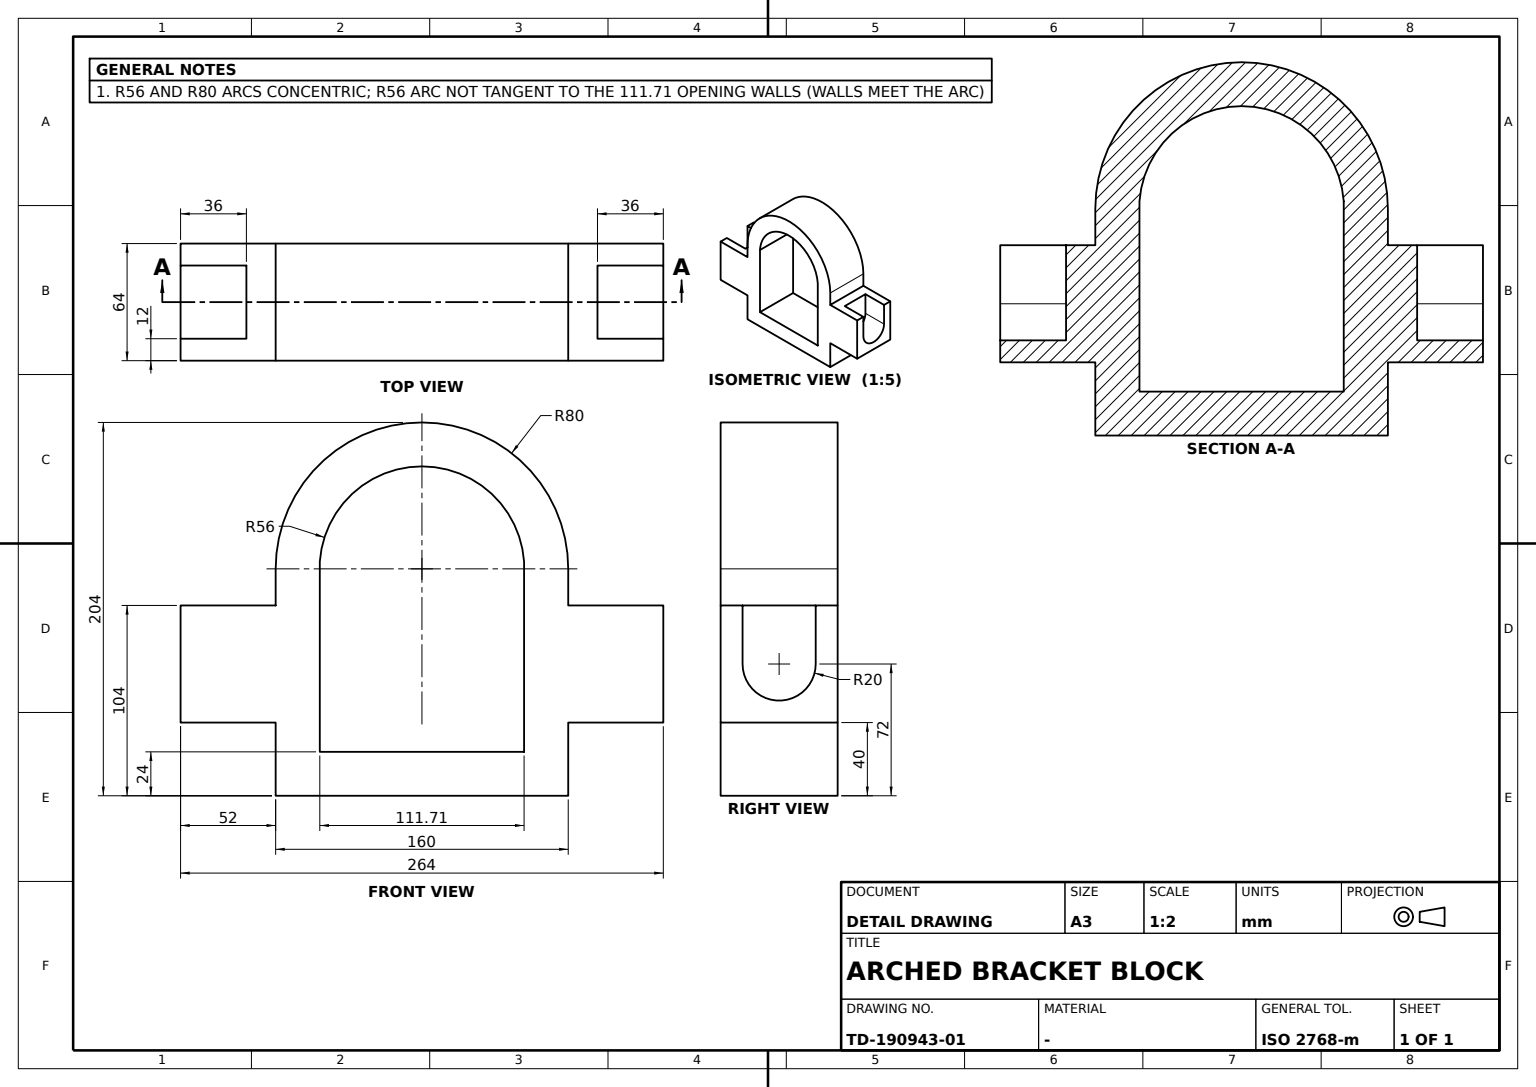
ISO-10303-21;
HEADER;
FILE_DESCRIPTION((''),'2;1');
FILE_NAME('','',(''),(''),'','','');
FILE_SCHEMA(('AUTOMOTIVE_DESIGN'));
ENDSEC;
DATA;
#1=APPLICATION_CONTEXT('');
#2=PRODUCT_CONTEXT('',#1,'mechanical');
#3=PRODUCT('','','',(#2));
#4=PRODUCT_DEFINITION_FORMATION('','',#3);
#5=PRODUCT_DEFINITION_CONTEXT('',#1,'design');
#6=PRODUCT_DEFINITION('','',#4,#5);
#7=PRODUCT_DEFINITION_SHAPE('','',#6);
#8=(LENGTH_UNIT()NAMED_UNIT(*)SI_UNIT(.MILLI.,.METRE.));
#9=(NAMED_UNIT(*)PLANE_ANGLE_UNIT()SI_UNIT($,.RADIAN.));
#10=(NAMED_UNIT(*)SI_UNIT($,.STERADIAN.)SOLID_ANGLE_UNIT());
#11=UNCERTAINTY_MEASURE_WITH_UNIT(LENGTH_MEASURE(0.005),#8,'distance_accuracy_value','');
#12=(GEOMETRIC_REPRESENTATION_CONTEXT(3)GLOBAL_UNCERTAINTY_ASSIGNED_CONTEXT((#11))GLOBAL_UNIT_ASSIGNED_CONTEXT((#8,#9,#10))REPRESENTATION_CONTEXT('',''));
#13=CARTESIAN_POINT('',(20.,-96.,-52.));
#14=VERTEX_POINT('',#13);
#15=CARTESIAN_POINT('',(-20.,-96.,-52.));
#16=VERTEX_POINT('',#15);
#17=CARTESIAN_POINT('',(0.,-96.,-52.));
#18=DIRECTION('',(0.,1.,0.));
#19=DIRECTION('',(0.,0.,1.));
#20=AXIS2_PLACEMENT_3D('',#17,#18,#19);
#21=CIRCLE('',#20,20.);
#22=EDGE_CURVE('',#14,#16,#21,.T.);
#23=ORIENTED_EDGE('',*,*,#22,.T.);
#24=CARTESIAN_POINT('',(-20.,-132.,-52.));
#25=VERTEX_POINT('',#24);
#26=CARTESIAN_POINT('',(-20.,114.,-52.));
#27=VECTOR('',#18,1000.);
#28=LINE('',#26,#27);
#29=EDGE_CURVE('',#25,#16,#28,.T.);
#30=ORIENTED_EDGE('',*,*,#29,.F.);
#31=CARTESIAN_POINT('',(20.,-132.,-52.));
#32=VERTEX_POINT('',#31);
#33=CARTESIAN_POINT('',(0.,-132.,-52.));
#34=DIRECTION('',(0.,-1.,0.));
#35=DIRECTION('',(0.,0.,-1.));
#36=AXIS2_PLACEMENT_3D('',#33,#34,#35);
#37=CIRCLE('',#36,20.);
#38=EDGE_CURVE('',#32,#25,#37,.F.);
#39=ORIENTED_EDGE('',*,*,#38,.F.);
#40=CARTESIAN_POINT('',(20.,114.,-52.));
#41=LINE('',#40,#27);
#42=EDGE_CURVE('',#32,#14,#41,.T.);
#43=ORIENTED_EDGE('',*,*,#42,.T.);
#44=EDGE_LOOP('',(#23,#30,#39,#43));
#45=FACE_BOUND('',#44,.T.);
#46=CARTESIAN_POINT('',(0.,114.,-52.));
#47=DIRECTION('',(-1.,0.,0.));
#48=AXIS2_PLACEMENT_3D('',#46,#18,#47);
#49=CYLINDRICAL_SURFACE('',#48,20.);
#50=ADVANCED_FACE('',(#45),#49,.F.);
#51=CARTESIAN_POINT('',(32.,132.,-84.));
#52=VERTEX_POINT('',#51);
#53=CARTESIAN_POINT('',(32.,80.,-84.));
#54=VERTEX_POINT('',#53);
#55=CARTESIAN_POINT('',(32.,-132.,-84.));
#56=VECTOR('',#34,1000.);
#57=LINE('',#55,#56);
#58=EDGE_CURVE('',#52,#54,#57,.T.);
#59=ORIENTED_EDGE('',*,*,#58,.T.);
#60=CARTESIAN_POINT('',(-32.,80.,-84.));
#61=VERTEX_POINT('',#60);
#62=CARTESIAN_POINT('',(0.,80.,-84.));
#63=DIRECTION('',(1.,0.,0.));
#64=VECTOR('',#63,1000.);
#65=LINE('',#62,#64);
#66=EDGE_CURVE('',#61,#54,#65,.T.);
#67=ORIENTED_EDGE('',*,*,#66,.F.);
#68=CARTESIAN_POINT('',(-32.,132.,-84.));
#69=VERTEX_POINT('',#68);
#70=CARTESIAN_POINT('',(-32.,-132.,-84.));
#71=LINE('',#70,#56);
#72=EDGE_CURVE('',#69,#61,#71,.T.);
#73=ORIENTED_EDGE('',*,*,#72,.F.);
#74=CARTESIAN_POINT('',(0.,132.,-84.));
#75=LINE('',#74,#64);
#76=EDGE_CURVE('',#69,#52,#75,.T.);
#77=ORIENTED_EDGE('',*,*,#76,.T.);
#78=EDGE_LOOP('',(#59,#67,#73,#77));
#79=FACE_BOUND('',#78,.T.);
#80=CARTESIAN_POINT('',(0.,-132.,-84.));
#81=AXIS2_PLACEMENT_3D('',#80,#35,#18);
#82=PLANE('',#81);
#83=ADVANCED_FACE('',(#79),#82,.T.);
#84=CARTESIAN_POINT('',(-32.,-80.,-84.));
#85=VERTEX_POINT('',#84);
#86=CARTESIAN_POINT('',(-32.,-80.,-124.));
#87=VERTEX_POINT('',#86);
#88=CARTESIAN_POINT('',(-32.,-80.,0.));
#89=VECTOR('',#35,1000.);
#90=LINE('',#88,#89);
#91=EDGE_CURVE('',#85,#87,#90,.T.);
#92=ORIENTED_EDGE('',*,*,#91,.T.);
#93=CARTESIAN_POINT('',(32.,-80.,-124.));
#94=VERTEX_POINT('',#93);
#95=CARTESIAN_POINT('',(0.,-80.,-124.));
#96=LINE('',#95,#64);
#97=EDGE_CURVE('',#87,#94,#96,.T.);
#98=ORIENTED_EDGE('',*,*,#97,.T.);
#99=CARTESIAN_POINT('',(32.,-80.,-84.));
#100=VERTEX_POINT('',#99);
#101=CARTESIAN_POINT('',(32.,-80.,0.));
#102=LINE('',#101,#89);
#103=EDGE_CURVE('',#100,#94,#102,.T.);
#104=ORIENTED_EDGE('',*,*,#103,.F.);
#105=CARTESIAN_POINT('',(0.,-80.,-84.));
#106=LINE('',#105,#64);
#107=EDGE_CURVE('',#85,#100,#106,.T.);
#108=ORIENTED_EDGE('',*,*,#107,.F.);
#109=EDGE_LOOP('',(#92,#98,#104,#108));
#110=FACE_BOUND('',#109,.T.);
#111=CARTESIAN_POINT('',(0.,-80.,0.));
#112=AXIS2_PLACEMENT_3D('',#111,#34,#35);
#113=PLANE('',#112);
#114=ADVANCED_FACE('',(#110),#113,.T.);
#115=CARTESIAN_POINT('',(20.,96.,-52.));
#116=VERTEX_POINT('',#115);
#117=CARTESIAN_POINT('',(-20.,96.,-52.));
#118=VERTEX_POINT('',#117);
#119=CARTESIAN_POINT('',(0.,96.,-52.));
#120=AXIS2_PLACEMENT_3D('',#119,#18,#19);
#121=CIRCLE('',#120,20.);
#122=EDGE_CURVE('',#116,#118,#121,.T.);
#123=ORIENTED_EDGE('',*,*,#122,.F.);
#124=CARTESIAN_POINT('',(20.,132.,-52.));
#125=VERTEX_POINT('',#124);
#126=EDGE_CURVE('',#125,#116,#41,.F.);
#127=ORIENTED_EDGE('',*,*,#126,.F.);
#128=CARTESIAN_POINT('',(-20.,132.,-52.));
#129=VERTEX_POINT('',#128);
#130=CARTESIAN_POINT('',(0.,132.,-52.));
#131=AXIS2_PLACEMENT_3D('',#130,#34,#35);
#132=CIRCLE('',#131,20.);
#133=EDGE_CURVE('',#125,#129,#132,.F.);
#134=ORIENTED_EDGE('',*,*,#133,.T.);
#135=EDGE_CURVE('',#129,#118,#28,.F.);
#136=ORIENTED_EDGE('',*,*,#135,.T.);
#137=EDGE_LOOP('',(#123,#127,#134,#136));
#138=FACE_BOUND('',#137,.T.);
#139=ADVANCED_FACE('',(#138),#49,.F.);
#140=ORIENTED_EDGE('',*,*,#126,.T.);
#141=CARTESIAN_POINT('',(20.,96.,-20.));
#142=VERTEX_POINT('',#141);
#143=LINE('',#141,#89);
#144=EDGE_CURVE('',#142,#116,#143,.T.);
#145=ORIENTED_EDGE('',*,*,#144,.F.);
#146=CARTESIAN_POINT('',(20.,132.,-20.));
#147=VERTEX_POINT('',#146);
#148=CARTESIAN_POINT('',(20.,-80.,-20.));
#149=LINE('',#148,#56);
#150=EDGE_CURVE('',#147,#142,#149,.T.);
#151=ORIENTED_EDGE('',*,*,#150,.F.);
#152=LINE('',#146,#89);
#153=EDGE_CURVE('',#147,#125,#152,.T.);
#154=ORIENTED_EDGE('',*,*,#153,.T.);
#155=EDGE_LOOP('',(#140,#145,#151,#154));
#156=FACE_BOUND('',#155,.T.);
#157=AXIS2_PLACEMENT_3D('',#146,#47,#35);
#158=PLANE('',#157);
#159=ADVANCED_FACE('',(#156),#158,.T.);
#160=CARTESIAN_POINT('',(-32.,55.85696,-100.));
#161=VERTEX_POINT('',#160);
#162=CARTESIAN_POINT('',(32.,55.85696,-100.));
#163=VERTEX_POINT('',#162);
#164=CARTESIAN_POINT('',(0.,55.85696,-100.));
#165=LINE('',#164,#64);
#166=EDGE_CURVE('',#161,#163,#165,.T.);
#167=ORIENTED_EDGE('',*,*,#166,.F.);
#168=CARTESIAN_POINT('',(-32.,-55.85696,-100.));
#169=VERTEX_POINT('',#168);
#170=CARTESIAN_POINT('',(-32.,0.,-100.));
#171=LINE('',#170,#27);
#172=EDGE_CURVE('',#169,#161,#171,.T.);
#173=ORIENTED_EDGE('',*,*,#172,.F.);
#174=CARTESIAN_POINT('',(32.,-55.85696,-100.));
#175=VERTEX_POINT('',#174);
#176=CARTESIAN_POINT('',(0.,-55.85696,-100.));
#177=LINE('',#176,#64);
#178=EDGE_CURVE('',#169,#175,#177,.T.);
#179=ORIENTED_EDGE('',*,*,#178,.T.);
#180=CARTESIAN_POINT('',(32.,0.,-100.));
#181=LINE('',#180,#27);
#182=EDGE_CURVE('',#175,#163,#181,.T.);
#183=ORIENTED_EDGE('',*,*,#182,.T.);
#184=EDGE_LOOP('',(#167,#173,#179,#183));
#185=FACE_BOUND('',#184,.T.);
#186=AXIS2_PLACEMENT_3D('',#176,#35,#18);
#187=PLANE('',#186);
#188=ADVANCED_FACE('',(#185),#187,.F.);
#189=CARTESIAN_POINT('',(-20.,132.,-20.));
#190=VERTEX_POINT('',#189);
#191=VECTOR('',#19,1000.);
#192=LINE('',#189,#191);
#193=EDGE_CURVE('',#129,#190,#192,.T.);
#194=ORIENTED_EDGE('',*,*,#193,.T.);
#195=CARTESIAN_POINT('',(-20.,96.,-20.));
#196=VERTEX_POINT('',#195);
#197=LINE('',#189,#56);
#198=EDGE_CURVE('',#190,#196,#197,.T.);
#199=ORIENTED_EDGE('',*,*,#198,.T.);
#200=LINE('',#117,#191);
#201=EDGE_CURVE('',#118,#196,#200,.T.);
#202=ORIENTED_EDGE('',*,*,#201,.F.);
#203=ORIENTED_EDGE('',*,*,#135,.F.);
#204=EDGE_LOOP('',(#194,#199,#202,#203));
#205=FACE_BOUND('',#204,.T.);
#206=AXIS2_PLACEMENT_3D('',#128,#63,#19);
#207=PLANE('',#206);
#208=ADVANCED_FACE('',(#205),#207,.T.);
#209=CARTESIAN_POINT('',(20.,-132.,-20.));
#210=VERTEX_POINT('',#209);
#211=CARTESIAN_POINT('',(32.,-132.,-20.));
#212=VERTEX_POINT('',#211);
#213=CARTESIAN_POINT('',(0.,-132.,-20.));
#214=LINE('',#213,#64);
#215=EDGE_CURVE('',#210,#212,#214,.T.);
#216=ORIENTED_EDGE('',*,*,#215,.F.);
#217=LINE('',#209,#89);
#218=EDGE_CURVE('',#210,#32,#217,.T.);
#219=ORIENTED_EDGE('',*,*,#218,.T.);
#220=ORIENTED_EDGE('',*,*,#38,.T.);
#221=CARTESIAN_POINT('',(-20.,-132.,-20.));
#222=VERTEX_POINT('',#221);
#223=LINE('',#221,#191);
#224=EDGE_CURVE('',#25,#222,#223,.T.);
#225=ORIENTED_EDGE('',*,*,#224,.T.);
#226=CARTESIAN_POINT('',(-32.,-132.,-20.));
#227=VERTEX_POINT('',#226);
#228=EDGE_CURVE('',#227,#222,#214,.T.);
#229=ORIENTED_EDGE('',*,*,#228,.F.);
#230=VERTEX_POINT('',#70);
#231=CARTESIAN_POINT('',(-32.,-132.,0.));
#232=LINE('',#231,#89);
#233=EDGE_CURVE('',#227,#230,#232,.T.);
#234=ORIENTED_EDGE('',*,*,#233,.T.);
#235=VERTEX_POINT('',#55);
#236=LINE('',#80,#64);
#237=EDGE_CURVE('',#230,#235,#236,.T.);
#238=ORIENTED_EDGE('',*,*,#237,.T.);
#239=CARTESIAN_POINT('',(32.,-132.,0.));
#240=LINE('',#239,#89);
#241=EDGE_CURVE('',#212,#235,#240,.T.);
#242=ORIENTED_EDGE('',*,*,#241,.F.);
#243=EDGE_LOOP('',(#216,#219,#220,#225,#229,#234,#238,#242));
#244=FACE_BOUND('',#243,.T.);
#245=AXIS2_PLACEMENT_3D('',#213,#34,#35);
#246=PLANE('',#245);
#247=ADVANCED_FACE('',(#244),#246,.T.);
#248=CARTESIAN_POINT('',(-32.,-80.,-20.));
#249=VERTEX_POINT('',#248);
#250=CARTESIAN_POINT('',(32.,-80.,-20.));
#251=VERTEX_POINT('',#250);
#252=CARTESIAN_POINT('',(0.,-80.,-20.));
#253=LINE('',#252,#64);
#254=EDGE_CURVE('',#249,#251,#253,.T.);
#255=ORIENTED_EDGE('',*,*,#254,.T.);
#256=VERTEX_POINT('',#101);
#257=EDGE_CURVE('',#256,#251,#102,.T.);
#258=ORIENTED_EDGE('',*,*,#257,.F.);
#259=VERTEX_POINT('',#88);
#260=LINE('',#111,#64);
#261=EDGE_CURVE('',#259,#256,#260,.T.);
#262=ORIENTED_EDGE('',*,*,#261,.F.);
#263=EDGE_CURVE('',#259,#249,#90,.T.);
#264=ORIENTED_EDGE('',*,*,#263,.T.);
#265=EDGE_LOOP('',(#255,#258,#262,#264));
#266=FACE_BOUND('',#265,.T.);
#267=ADVANCED_FACE('',(#266),#113,.T.);
#268=CARTESIAN_POINT('',(-32.,80.,0.));
#269=VERTEX_POINT('',#268);
#270=CARTESIAN_POINT('',(-32.,0.,0.));
#271=AXIS2_PLACEMENT_3D('',#270,#63,#35);
#272=CIRCLE('',#271,80.);
#273=EDGE_CURVE('',#269,#259,#272,.T.);
#274=ORIENTED_EDGE('',*,*,#273,.T.);
#275=ORIENTED_EDGE('',*,*,#261,.T.);
#276=CARTESIAN_POINT('',(32.,80.,0.));
#277=VERTEX_POINT('',#276);
#278=CARTESIAN_POINT('',(32.,0.,0.));
#279=AXIS2_PLACEMENT_3D('',#278,#63,#35);
#280=CIRCLE('',#279,80.);
#281=EDGE_CURVE('',#277,#256,#280,.T.);
#282=ORIENTED_EDGE('',*,*,#281,.F.);
#283=CARTESIAN_POINT('',(0.,80.,0.));
#284=LINE('',#283,#64);
#285=EDGE_CURVE('',#269,#277,#284,.T.);
#286=ORIENTED_EDGE('',*,*,#285,.F.);
#287=EDGE_LOOP('',(#274,#275,#282,#286));
#288=FACE_BOUND('',#287,.T.);
#289=CARTESIAN_POINT('',(0.,0.,0.));
#290=AXIS2_PLACEMENT_3D('',#289,#63,#18);
#291=CYLINDRICAL_SURFACE('',#290,80.);
#292=ADVANCED_FACE('',(#288),#291,.T.);
#293=CARTESIAN_POINT('',(-32.,80.,-20.));
#294=VERTEX_POINT('',#293);
#295=CARTESIAN_POINT('',(-32.,132.,-20.));
#296=VERTEX_POINT('',#295);
#297=LINE('',#248,#27);
#298=EDGE_CURVE('',#294,#296,#297,.T.);
#299=ORIENTED_EDGE('',*,*,#298,.F.);
#300=CARTESIAN_POINT('',(32.,80.,-20.));
#301=VERTEX_POINT('',#300);
#302=CARTESIAN_POINT('',(0.,80.,-20.));
#303=LINE('',#302,#64);
#304=EDGE_CURVE('',#294,#301,#303,.T.);
#305=ORIENTED_EDGE('',*,*,#304,.T.);
#306=CARTESIAN_POINT('',(32.,132.,-20.));
#307=VERTEX_POINT('',#306);
#308=LINE('',#250,#27);
#309=EDGE_CURVE('',#301,#307,#308,.T.);
#310=ORIENTED_EDGE('',*,*,#309,.T.);
#311=CARTESIAN_POINT('',(0.,132.,-20.));
#312=LINE('',#311,#64);
#313=EDGE_CURVE('',#147,#307,#312,.T.);
#314=ORIENTED_EDGE('',*,*,#313,.F.);
#315=ORIENTED_EDGE('',*,*,#150,.T.);
#316=CARTESIAN_POINT('',(0.,96.,-20.));
#317=LINE('',#316,#64);
#318=EDGE_CURVE('',#196,#142,#317,.T.);
#319=ORIENTED_EDGE('',*,*,#318,.F.);
#320=ORIENTED_EDGE('',*,*,#198,.F.);
#321=EDGE_CURVE('',#296,#190,#312,.T.);
#322=ORIENTED_EDGE('',*,*,#321,.F.);
#323=EDGE_LOOP('',(#299,#305,#310,#314,#315,#319,#320,#322));
#324=FACE_BOUND('',#323,.T.);
#325=AXIS2_PLACEMENT_3D('',#252,#19,#34);
#326=PLANE('',#325);
#327=ADVANCED_FACE('',(#324),#326,.T.);
#328=ORIENTED_EDGE('',*,*,#22,.F.);
#329=CARTESIAN_POINT('',(20.,-96.,-20.));
#330=VERTEX_POINT('',#329);
#331=LINE('',#329,#89);
#332=EDGE_CURVE('',#330,#14,#331,.T.);
#333=ORIENTED_EDGE('',*,*,#332,.F.);
#334=CARTESIAN_POINT('',(-20.,-96.,-20.));
#335=VERTEX_POINT('',#334);
#336=CARTESIAN_POINT('',(0.,-96.,-20.));
#337=LINE('',#336,#64);
#338=EDGE_CURVE('',#335,#330,#337,.T.);
#339=ORIENTED_EDGE('',*,*,#338,.F.);
#340=LINE('',#15,#191);
#341=EDGE_CURVE('',#16,#335,#340,.T.);
#342=ORIENTED_EDGE('',*,*,#341,.F.);
#343=EDGE_LOOP('',(#328,#333,#339,#342));
#344=FACE_BOUND('',#343,.T.);
#345=CARTESIAN_POINT('',(0.,-96.,0.));
#346=AXIS2_PLACEMENT_3D('',#345,#18,#47);
#347=PLANE('',#346);
#348=ADVANCED_FACE('',(#344),#347,.F.);
#349=ORIENTED_EDGE('',*,*,#42,.F.);
#350=ORIENTED_EDGE('',*,*,#218,.F.);
#351=LINE('',#146,#27);
#352=EDGE_CURVE('',#210,#330,#351,.T.);
#353=ORIENTED_EDGE('',*,*,#352,.T.);
#354=ORIENTED_EDGE('',*,*,#332,.T.);
#355=EDGE_LOOP('',(#349,#350,#353,#354));
#356=FACE_BOUND('',#355,.T.);
#357=ADVANCED_FACE('',(#356),#158,.T.);
#358=CARTESIAN_POINT('',(32.,80.,-124.));
#359=VERTEX_POINT('',#358);
#360=LINE('',#276,#191);
#361=EDGE_CURVE('',#359,#54,#360,.T.);
#362=ORIENTED_EDGE('',*,*,#361,.F.);
#363=CARTESIAN_POINT('',(-32.,80.,-124.));
#364=VERTEX_POINT('',#363);
#365=CARTESIAN_POINT('',(0.,80.,-124.));
#366=LINE('',#365,#64);
#367=EDGE_CURVE('',#364,#359,#366,.T.);
#368=ORIENTED_EDGE('',*,*,#367,.F.);
#369=LINE('',#268,#191);
#370=EDGE_CURVE('',#364,#61,#369,.T.);
#371=ORIENTED_EDGE('',*,*,#370,.T.);
#372=ORIENTED_EDGE('',*,*,#66,.T.);
#373=EDGE_LOOP('',(#362,#368,#371,#372));
#374=FACE_BOUND('',#373,.T.);
#375=AXIS2_PLACEMENT_3D('',#365,#18,#19);
#376=PLANE('',#375);
#377=ADVANCED_FACE('',(#374),#376,.T.);
#378=CARTESIAN_POINT('',(-32.,55.85696,4.));
#379=VERTEX_POINT('',#378);
#380=CARTESIAN_POINT('',(32.,55.85696,4.));
#381=VERTEX_POINT('',#380);
#382=LINE('',#378,#64);
#383=EDGE_CURVE('',#379,#381,#382,.T.);
#384=ORIENTED_EDGE('',*,*,#383,.F.);
#385=CARTESIAN_POINT('',(-32.,55.85696,0.));
#386=LINE('',#385,#191);
#387=EDGE_CURVE('',#161,#379,#386,.T.);
#388=ORIENTED_EDGE('',*,*,#387,.F.);
#389=ORIENTED_EDGE('',*,*,#166,.T.);
#390=CARTESIAN_POINT('',(32.,55.85696,0.));
#391=LINE('',#390,#191);
#392=EDGE_CURVE('',#163,#381,#391,.T.);
#393=ORIENTED_EDGE('',*,*,#392,.T.);
#394=EDGE_LOOP('',(#384,#388,#389,#393));
#395=FACE_BOUND('',#394,.T.);
#396=AXIS2_PLACEMENT_3D('',#164,#18,#19);
#397=PLANE('',#396);
#398=ADVANCED_FACE('',(#395),#397,.F.);
#399=ORIENTED_EDGE('',*,*,#309,.F.);
#400=EDGE_CURVE('',#301,#277,#360,.T.);
#401=ORIENTED_EDGE('',*,*,#400,.T.);
#402=ORIENTED_EDGE('',*,*,#281,.T.);
#403=ORIENTED_EDGE('',*,*,#257,.T.);
#404=CARTESIAN_POINT('',(32.,0.,-20.));
#405=LINE('',#404,#56);
#406=EDGE_CURVE('',#251,#212,#405,.T.);
#407=ORIENTED_EDGE('',*,*,#406,.T.);
#408=ORIENTED_EDGE('',*,*,#241,.T.);
#409=CARTESIAN_POINT('',(32.,0.,-84.));
#410=LINE('',#409,#27);
#411=EDGE_CURVE('',#235,#100,#410,.T.);
#412=ORIENTED_EDGE('',*,*,#411,.T.);
#413=ORIENTED_EDGE('',*,*,#103,.T.);
#414=CARTESIAN_POINT('',(32.,0.,-124.));
#415=LINE('',#414,#27);
#416=EDGE_CURVE('',#94,#359,#415,.T.);
#417=ORIENTED_EDGE('',*,*,#416,.T.);
#418=ORIENTED_EDGE('',*,*,#361,.T.);
#419=ORIENTED_EDGE('',*,*,#58,.F.);
#420=CARTESIAN_POINT('',(32.,132.,0.));
#421=LINE('',#420,#89);
#422=EDGE_CURVE('',#307,#52,#421,.T.);
#423=ORIENTED_EDGE('',*,*,#422,.F.);
#424=EDGE_LOOP('',(#399,#401,#402,#403,#407,#408,#412,#413,#417,#418,#419,#423));
#425=FACE_BOUND('',#424,.T.);
#426=ORIENTED_EDGE('',*,*,#182,.F.);
#427=CARTESIAN_POINT('',(32.,-55.85696,4.));
#428=VERTEX_POINT('',#427);
#429=CARTESIAN_POINT('',(32.,-55.85696,0.));
#430=LINE('',#429,#89);
#431=EDGE_CURVE('',#428,#175,#430,.T.);
#432=ORIENTED_EDGE('',*,*,#431,.F.);
#433=CIRCLE('',#279,56.);
#434=EDGE_CURVE('',#381,#428,#433,.T.);
#435=ORIENTED_EDGE('',*,*,#434,.F.);
#436=ORIENTED_EDGE('',*,*,#392,.F.);
#437=EDGE_LOOP('',(#426,#432,#435,#436));
#438=FACE_BOUND('',#437,.T.);
#439=AXIS2_PLACEMENT_3D('',#278,#63,#18);
#440=PLANE('',#439);
#441=ADVANCED_FACE('',(#425,#438),#440,.T.);
#442=ORIENTED_EDGE('',*,*,#107,.T.);
#443=ORIENTED_EDGE('',*,*,#411,.F.);
#444=ORIENTED_EDGE('',*,*,#237,.F.);
#445=CARTESIAN_POINT('',(-32.,0.,-84.));
#446=LINE('',#445,#27);
#447=EDGE_CURVE('',#230,#85,#446,.T.);
#448=ORIENTED_EDGE('',*,*,#447,.T.);
#449=EDGE_LOOP('',(#442,#443,#444,#448));
#450=FACE_BOUND('',#449,.T.);
#451=ADVANCED_FACE('',(#450),#82,.T.);
#452=ORIENTED_EDGE('',*,*,#383,.T.);
#453=ORIENTED_EDGE('',*,*,#434,.T.);
#454=CARTESIAN_POINT('',(-32.,-55.85696,4.));
#455=VERTEX_POINT('',#454);
#456=LINE('',#454,#64);
#457=EDGE_CURVE('',#455,#428,#456,.T.);
#458=ORIENTED_EDGE('',*,*,#457,.F.);
#459=CIRCLE('',#271,56.);
#460=EDGE_CURVE('',#379,#455,#459,.T.);
#461=ORIENTED_EDGE('',*,*,#460,.F.);
#462=EDGE_LOOP('',(#452,#453,#458,#461));
#463=FACE_BOUND('',#462,.T.);
#464=CYLINDRICAL_SURFACE('',#290,56.);
#465=ADVANCED_FACE('',(#463),#464,.F.);
#466=ORIENTED_EDGE('',*,*,#228,.T.);
#467=CARTESIAN_POINT('',(-20.,-80.,-20.));
#468=LINE('',#467,#27);
#469=EDGE_CURVE('',#222,#335,#468,.T.);
#470=ORIENTED_EDGE('',*,*,#469,.T.);
#471=ORIENTED_EDGE('',*,*,#338,.T.);
#472=ORIENTED_EDGE('',*,*,#352,.F.);
#473=ORIENTED_EDGE('',*,*,#215,.T.);
#474=ORIENTED_EDGE('',*,*,#406,.F.);
#475=ORIENTED_EDGE('',*,*,#254,.F.);
#476=CARTESIAN_POINT('',(-32.,0.,-20.));
#477=LINE('',#476,#56);
#478=EDGE_CURVE('',#249,#227,#477,.T.);
#479=ORIENTED_EDGE('',*,*,#478,.T.);
#480=EDGE_LOOP('',(#466,#470,#471,#472,#473,#474,#475,#479));
#481=FACE_BOUND('',#480,.T.);
#482=ADVANCED_FACE('',(#481),#326,.T.);
#483=ORIENTED_EDGE('',*,*,#431,.T.);
#484=ORIENTED_EDGE('',*,*,#178,.F.);
#485=CARTESIAN_POINT('',(-32.,-55.85696,0.));
#486=LINE('',#485,#89);
#487=EDGE_CURVE('',#455,#169,#486,.T.);
#488=ORIENTED_EDGE('',*,*,#487,.F.);
#489=ORIENTED_EDGE('',*,*,#457,.T.);
#490=EDGE_LOOP('',(#483,#484,#488,#489));
#491=FACE_BOUND('',#490,.T.);
#492=CARTESIAN_POINT('',(0.,-55.85696,4.));
#493=AXIS2_PLACEMENT_3D('',#492,#34,#35);
#494=PLANE('',#493);
#495=ADVANCED_FACE('',(#491),#494,.F.);
#496=ORIENTED_EDGE('',*,*,#285,.T.);
#497=ORIENTED_EDGE('',*,*,#400,.F.);
#498=ORIENTED_EDGE('',*,*,#304,.F.);
#499=EDGE_CURVE('',#294,#269,#369,.T.);
#500=ORIENTED_EDGE('',*,*,#499,.T.);
#501=EDGE_LOOP('',(#496,#497,#498,#500));
#502=FACE_BOUND('',#501,.T.);
#503=ADVANCED_FACE('',(#502),#376,.T.);
#504=CARTESIAN_POINT('',(-32.,132.,0.));
#505=LINE('',#504,#89);
#506=EDGE_CURVE('',#296,#69,#505,.T.);
#507=ORIENTED_EDGE('',*,*,#506,.F.);
#508=ORIENTED_EDGE('',*,*,#321,.T.);
#509=ORIENTED_EDGE('',*,*,#193,.F.);
#510=ORIENTED_EDGE('',*,*,#133,.F.);
#511=ORIENTED_EDGE('',*,*,#153,.F.);
#512=ORIENTED_EDGE('',*,*,#313,.T.);
#513=ORIENTED_EDGE('',*,*,#422,.T.);
#514=ORIENTED_EDGE('',*,*,#76,.F.);
#515=EDGE_LOOP('',(#507,#508,#509,#510,#511,#512,#513,#514));
#516=FACE_BOUND('',#515,.T.);
#517=AXIS2_PLACEMENT_3D('',#311,#34,#35);
#518=PLANE('',#517);
#519=ADVANCED_FACE('',(#516),#518,.F.);
#520=ORIENTED_EDGE('',*,*,#144,.T.);
#521=ORIENTED_EDGE('',*,*,#122,.T.);
#522=ORIENTED_EDGE('',*,*,#201,.T.);
#523=ORIENTED_EDGE('',*,*,#318,.T.);
#524=EDGE_LOOP('',(#520,#521,#522,#523));
#525=FACE_BOUND('',#524,.T.);
#526=CARTESIAN_POINT('',(0.,96.,0.));
#527=AXIS2_PLACEMENT_3D('',#526,#18,#47);
#528=PLANE('',#527);
#529=ADVANCED_FACE('',(#525),#528,.T.);
#530=ORIENTED_EDGE('',*,*,#506,.T.);
#531=ORIENTED_EDGE('',*,*,#72,.T.);
#532=ORIENTED_EDGE('',*,*,#370,.F.);
#533=CARTESIAN_POINT('',(-32.,0.,-124.));
#534=LINE('',#533,#27);
#535=EDGE_CURVE('',#87,#364,#534,.T.);
#536=ORIENTED_EDGE('',*,*,#535,.F.);
#537=ORIENTED_EDGE('',*,*,#91,.F.);
#538=ORIENTED_EDGE('',*,*,#447,.F.);
#539=ORIENTED_EDGE('',*,*,#233,.F.);
#540=ORIENTED_EDGE('',*,*,#478,.F.);
#541=ORIENTED_EDGE('',*,*,#263,.F.);
#542=ORIENTED_EDGE('',*,*,#273,.F.);
#543=ORIENTED_EDGE('',*,*,#499,.F.);
#544=ORIENTED_EDGE('',*,*,#298,.T.);
#545=EDGE_LOOP('',(#530,#531,#532,#536,#537,#538,#539,#540,#541,#542,#543,#544));
#546=FACE_BOUND('',#545,.T.);
#547=ORIENTED_EDGE('',*,*,#387,.T.);
#548=ORIENTED_EDGE('',*,*,#460,.T.);
#549=ORIENTED_EDGE('',*,*,#487,.T.);
#550=ORIENTED_EDGE('',*,*,#172,.T.);
#551=EDGE_LOOP('',(#547,#548,#549,#550));
#552=FACE_BOUND('',#551,.T.);
#553=AXIS2_PLACEMENT_3D('',#270,#63,#18);
#554=PLANE('',#553);
#555=ADVANCED_FACE('',(#546,#552),#554,.F.);
#556=ORIENTED_EDGE('',*,*,#97,.F.);
#557=ORIENTED_EDGE('',*,*,#535,.T.);
#558=ORIENTED_EDGE('',*,*,#367,.T.);
#559=ORIENTED_EDGE('',*,*,#416,.F.);
#560=EDGE_LOOP('',(#556,#557,#558,#559));
#561=FACE_BOUND('',#560,.T.);
#562=AXIS2_PLACEMENT_3D('',#95,#35,#18);
#563=PLANE('',#562);
#564=ADVANCED_FACE('',(#561),#563,.T.);
#565=ORIENTED_EDGE('',*,*,#29,.T.);
#566=ORIENTED_EDGE('',*,*,#341,.T.);
#567=ORIENTED_EDGE('',*,*,#469,.F.);
#568=ORIENTED_EDGE('',*,*,#224,.F.);
#569=EDGE_LOOP('',(#565,#566,#567,#568));
#570=FACE_BOUND('',#569,.T.);
#571=ADVANCED_FACE('',(#570),#207,.T.);
#572=CLOSED_SHELL('',(#50,#83,#114,#139,#159,#188,#208,#247,#267,#292,#327,#348,#357,#377,#398,#441,#451,#465,#482,#495,#503,#519,#529,#555,#564,#571));
#573=MANIFOLD_SOLID_BREP('',#572);
#574=ADVANCED_BREP_SHAPE_REPRESENTATION('',(#573),#12);
#575=SHAPE_DEFINITION_REPRESENTATION(#7,#574);
ENDSEC;
END-ISO-10303-21;
